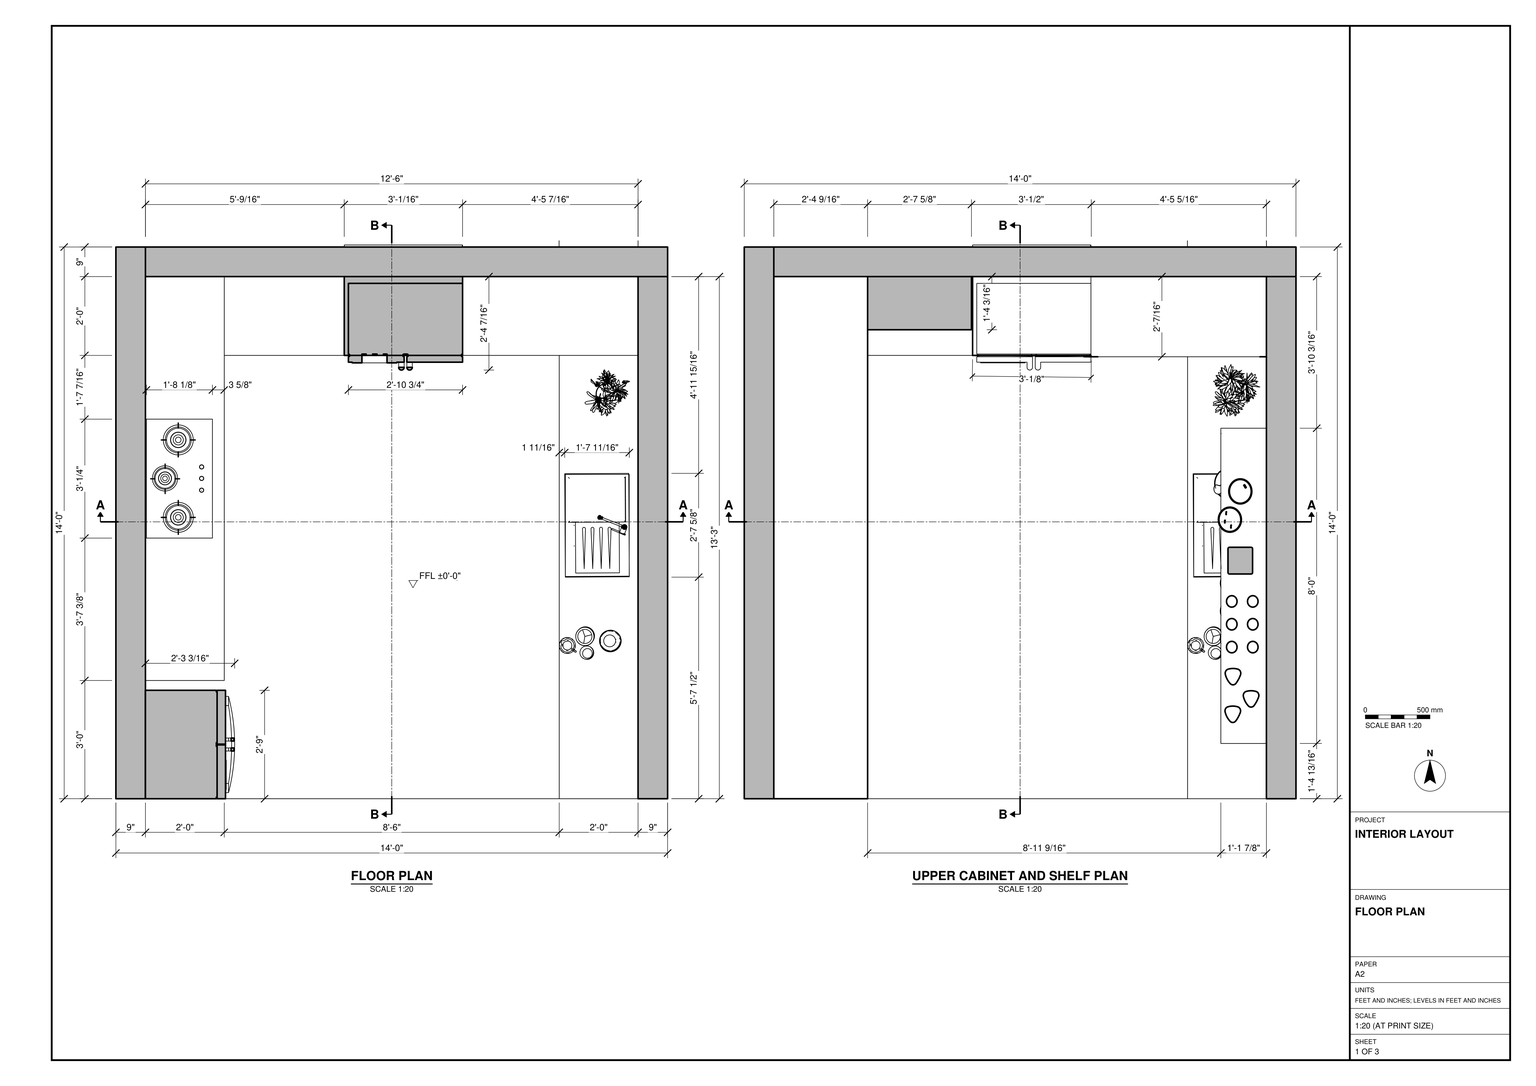
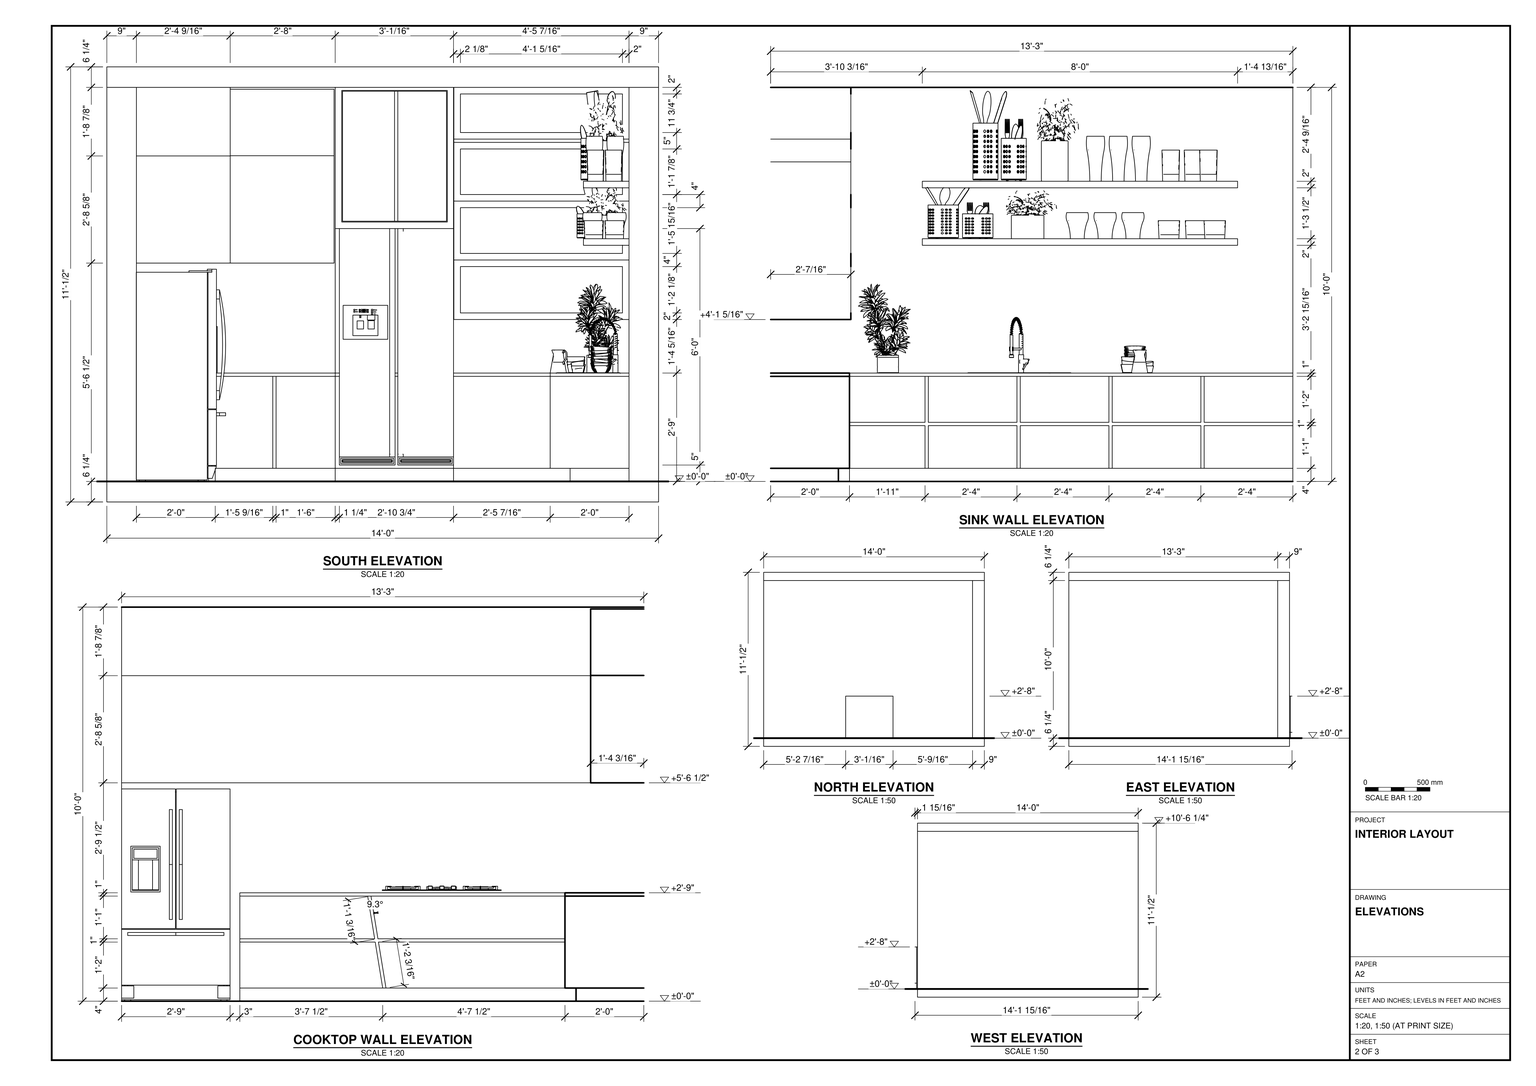
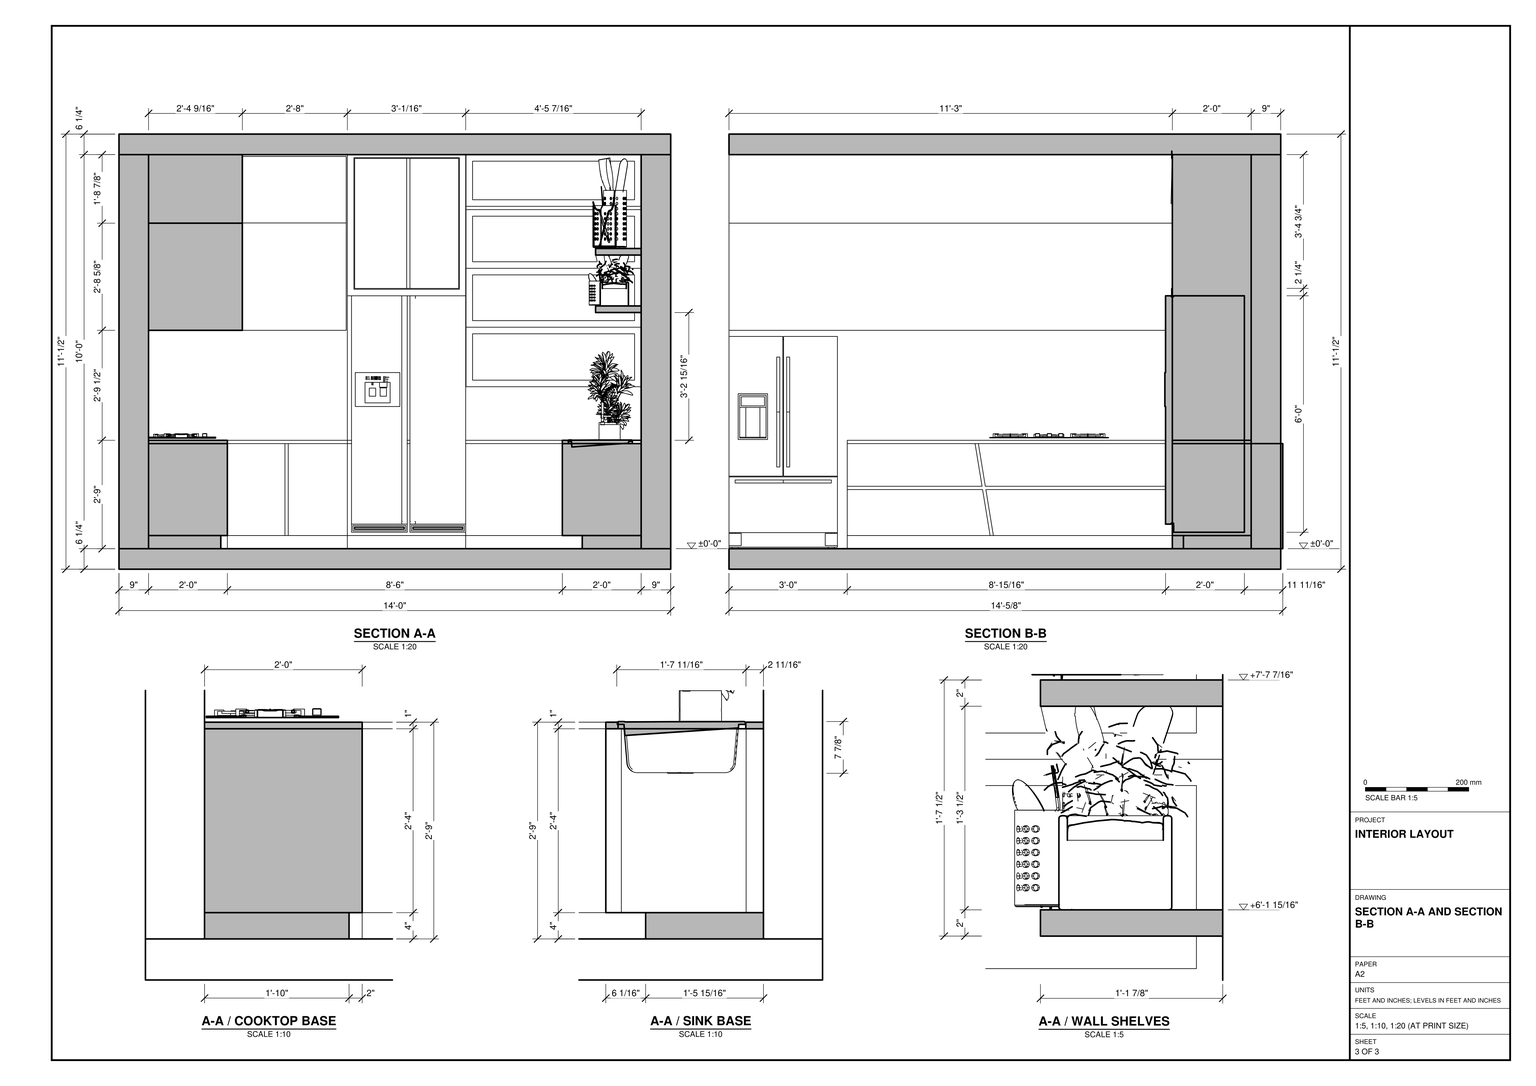
Build the kitchen interior shown in task_files/diagram_01.pdf. Work in feet and inches. The overall model is 14'-0" wide, 14'-5/8" deep and 11'-1/2" high, with a single finished floor level at ±0'-0". Model the floor and ceiling slabs and the 9" side and back walls, leaving the front open as drawn.

Use the floor plan to set out the cooktop run on the left and the sink run on the right, with 8'-6" clear between their counter edges. Use the elevations and section details to shape the worktops, recessed plinths and cabinet fronts. Include the sink, drainer and faucet. Place one refrigerator at the open end of the cooktop wall and the other in the back-wall cabinetry. Follow the upper cabinet and shelf plan for the overhead cupboards and the pair of long shelves above the sink counter. Decor and loose items, including plants, vessels and appliances, may be any suitable library components placed as shown.

Keep the walls and slabs and each piece of joinery or furniture in separate groups or components, and use components for repeated parts. Save one SketchUp model as output_files/kitchen_with_opposing_counters_and_wall_mounted_storage.skp.

# SketchUp Ruby script. Lengths in inches.
U = 1.inch
M = Sketchup.active_model
def pt(a) = Geom::Point3d.new(a.map { |v| v * U })
def face(e, loops, mat)
  f = e.add_face(loops[0].map { |a| pt(a) })
  loops[1..].each { |l| e.add_face(l.map { |a| pt(a) }).erase! }
  f.material = f.back_material = mat if mat
  f
end
# faces: each face lists its corners as indices into pts; further lists are holes
def faces(e, pts, list, mat = nil) = list.each { |f| face(e, (f[0].is_a?(Array) ? f : [f]).map { |l| l.map { |i| pts[i] } }, mat) }
# xy, xz, yz: faces in a plane at the given z, y or x. An outline is a flat list of corners, or four numbers for a rectangle; further outlines are holes
def ring(l) = l.size == 4 ? [[l[0], l[1]], [l[2], l[1]], [l[2], l[3]], [l[0], l[3]]] : l.each_slice(2).to_a
def flat(e, list, mat, &to3) = list.each { |f| face(e, (f[0].is_a?(Array) ? f : [f]).map { |l| ring(l).map { |u, v| to3.(u, v) } }, mat) }
def xy(e, z, list, mat = nil) = flat(e, list, mat) { |x, y| [x, y, z] }
def xz(e, y, list, mat = nil) = flat(e, list, mat) { |x, z| [x, y, z] }
def yz(e, x, list, mat = nil) = flat(e, list, mat) { |y, z| [x, y, z] }
def lines(e, pts, list) = list.each { |a, b| e.add_line(pt(pts[a]), pt(pts[b])) }
# prism: a flat outline (further loops are holes) pulled along v
def prism(e, loops, v, mat = nil)
  f = face(e, loops, mat); d = Geom::Vector3d.new(v.map { |x| x * U })
  f.pushpull(f.normal.samedirection?(d) ? d.length : -d.length)
end
def box(e, o, s, mat = nil) = prism(e, [[o, [o[0] + s[0], o[1], o[2]], [o[0] + s[0], o[1] + s[1], o[2]], [o[0], o[1] + s[1], o[2]]]], [0, 0, s[2]], mat)
def at(x, y, z, deg = 0) = Geom::Transformation.translation(pt([x, y, z])) * Geom::Transformation.rotation(ORIGIN, Z_AXIS, deg.degrees)
def axes(o, x, y, z) = Geom::Transformation.new([*x, 0, *y, 0, *z, 0, *pt(o).to_a, 1])
def part(name) = M.definitions.add(name)
# library, detail: a bought-in or finely detailed component or shape, given as its bounding box
def library(name, o, s) = part(name).tap { |d| box(d.entities, o, s) }
def detail(e, o, s) = box(e.add_group.entities, o, s)
def put(e, d, t, mat = nil) = e.add_instance(d, t).tap { |i| i.material = mat if mat }
def group(e, t, mat = nil) = e.add_group.tap { |g| g.transformation = t; g.material = mat if mat }.entities
root = M.entities
M.materials.add("[Concrete Tile]").color = [203, 190, 164]
M.materials.add("[Field Square Tile]").color = [217, 201, 169]
M.materials.add("[Marble Carrara Gold Floor Tile]").color = [225, 223, 217]
M.materials.add("[Tile Canvas]").color = [199, 192, 173]
M.materials.add("[Tile Ceramic Multi]").color = [165, 115, 84]
M.materials.add("[Wood Square Tile 01]").color = [164, 91, 44]
c1 = library("Fridge\#1",[0,-2.9,-33.83],[42,31.9,87])
c2 = library("French door refrigerator",[0,0,0],[35.5,29.25,69.5])
c3 = library("Kitchen sink",[0,0,0],[31.5,19.49,24.78])
c4 = library("plant",[-35.72,-28.42,0],[66.31,67.39,84.38])
c5 = library("Bosch Stove",[0,0,0],[36.22,20.12,1.38])
c6 = library("3",[-1.02,-0.875,0],[20.82,14.52,8.31])
c7 = library("cups",[-1.65,2.1875,0],[44.23,8.89,10.3125])
c8 = part("Difference")
prism(c8.entities,[[[24,135,0],[24,0,0],[0,0,0],[0,135,0]],[[1.87,67.61,0],[21.31,67.61,0],[21.31,98.77,0],[1.87,98.77,0]]],[0,0,1])
xy(root,6.25,[[69.53,135,105.57,139.0625]])
xy(root,10.25,[[137.36,73.95,156.36,104.95],[69.53,135,105.57,159]])
xy(root,55.5625,[[105.57,134.59,159,159]])
xy(root,78.16,[[145.125,16.82,159,112.82]])
xy(root,80.16,[[145.125,16.82,159,112.82]],"[Tile Ceramic Multi]")
xy(root,95.66,[[145.125,16.82,159,112.82]])
xy(root,97.66,[[145.125,16.82,159,112.82]],"[Tile Ceramic Multi]")
xy(root,126.25,[[105.57,134.59,159,159]])
xz(root,16.82,[[145.125,78.16,159,80.16],[145.125,95.66,159,97.66]])
xz(root,112.82,[[145.125,78.16,159,80.16],[145.125,95.66,159,97.66]])
xz(root,134.59,[[105.57,55.5625,105.67,126.25],[[105.67,55.5625,159,73.6875],[107.67,57.5625,157,71.6875]],[[105.67,73.6875,159,91.625],[107.67,75.6875,157,89.625]],[[105.67,91.625,159,109.5],[107.67,93.625,157,107.5]],[105.67,109.5,159,110.5],
  [[105.67,110.5,159,126.25],[107.67,112.5,157,124.25]]])
xz(root,135,[[69.53,6.25,105.57,10.25]])
xz(root,135,[[69.53,38.25,105.57,126.25]],"[Wood Square Tile 01]")
xz(root,159,[[105.57,55.5625,159,126.25]],"[Wood Square Tile 01]")
yz(root,69.53,[[135,10.25,159,126.25]])
yz(root,105.57,[[135,10.25,159,55.5625],[134.59,55.5625,135,126.25]])
yz(root,145.125,[[16.82,78.16,112.82,80.16],[16.82,95.66,112.82,97.66]])
yz(root,159,[[134.59,55.5625,159,103.5625],[16.82,78.16,112.82,80.16],[16.82,95.66,112.82,97.66],[134.59,103.5625,159,110.5],[134.59,110.5,159,126.25]])
p = [[105.67,134.59,127.32],[69.53,135,127.32],[69.53,135,126.25],[69.53,135,83.25],[105.67,134.59,83.25],[105.67,134.59,91.625],
  [105.67,134.59,109.5],[105.67,134.59,110.5],[105.67,134.59,126.25],[71.53,134.98,85.25],[71.53,134.98,125.32],[103.67,134.61,125.32],
  [103.67,134.61,110.5],[103.67,134.61,109.5],[103.67,134.61,91.625],[103.67,134.61,85.25],[71.77,134.97,85.5],[71.77,134.97,125.08],
  [87.6,134.79,125.08],[103.43,134.61,125.08],[103.43,134.61,85.5],[87.6,134.79,85.5],[159,169.92,38.25],[159,168,38.25],
  [134.95,168,10.69],[134.95,169.92,10.69],[69.53,139.0625,6.25],[69.53,139.0625,10.25],[105.57,139.0625,10.25],[105.57,139.0625,6.25],
  [135,28,38.25],[135,28,24.25],[135,56,38.25],[135,56,24.25],[135,84,38.25],[135,84,24.25],
  [135,112,38.25],[135,112,24.25],[50.54,135,38.25],[50.54,135,10.25],[135,0,24.25],[135,27,24.25],
  [135,55,24.25],[135,83,24.25],[135,111,24.25],[135,135,24.25],[69.53,134.59,111.25],[135,27,38.25],
  [135,55,38.25],[135,112,23.25],[135,135,23.25],[135,28,23.25],[135,55,23.25],[135,56,23.25],
  [135,83,23.25],[135,84,23.25],[135,111,23.25],[135,0,23.25],[135,27,23.25],[135,28,10.25],
  [135,56,10.25],[135,84,10.25],[135,112,10.25],[135,27,10.25],[135,55,10.25],[135,83,38.25],
  [135,83,10.25],[135,111,38.25],[135,111,10.25],[33,74.92,38.25],[33,77.05,25.25],[33,77.21,24.25],
  [33,79.5,10.25],[33,78.21,24.25],[33,80.5,10.25],[33,135,24.25],[33,78.21,25.25],[33,135,25.25],
  [33,75.92,38.25],[33,78.05,25.25],[33,31.57,25.25],[33,31.48,25.25],[51.54,135,38.25],[51.54,135,10.25],
  [88.6,134.79,125.08],[88.6,134.79,85.5],[33,36,24.25],[33,36,25.25],[156.36,104.95,39.25],[156.36,104.95,10.25],
  [156.36,73.95,39.25],[156.36,73.95,10.25],[137.36,104.95,39.25],[137.36,104.95,10.25],[137.36,73.95,39.25],[137.36,73.95,10.25]]
faces(root,p,[[[0,1,2,3,4,5,6,7,8],[9,10,11,12,13,14,15]],[[10,9,15,14,13,12,11],[16,17,18,19,20,21]]])
lines(root,p,[[22,23],[24,25],[26,27],[28,29],[30,31],[32,33],[34,35],[36,37],[38,39],[40,41],[31,42],[33,43],
  [35,44],[37,45],[46,1],[47,41],[48,42],[49,50],[51,52],[53,54],[55,56],[57,58],[51,59],[53,60],
  [55,61],[49,62],[58,63],[52,64],[65,43],[54,66],[67,44],[56,68],[69,70],[71,72],[73,74],[73,75],
  [76,77],[78,79],[76,79],[80,81],[82,83],[18,21],[84,85],[71,86],[70,87],[88,89],[90,91],[92,93],
  [94,95]])
put(root,c1,axes([70.8,132.93,39.25],[0.8277,0,0],[0,0.8277,0],[0,0,0.8277]))
put(root,c2,axes([8.96,33.01,6.25],[0,-0.93,0],[0.93,0,0],[0,0,0.93]))
put(root,c3,at(136.67,98.97,31.47,-89.672))
put(root,c4,axes([149.17,122.76,39.25],[0.3213,0,0],[0,0.3213,0],[0,0,0.3213]))
put(root,c5,at(29.4,79.37,39.95,90))
put(root,c6,at(135,41.36,39.25))
put(root,c7,axes([140.16,98.27,97.66],[0,-1.76715,0],[1.62497,0,0],[0,0,2.6775]))
put(root,c7,axes([138.34,112.14,80.16],[0,-2.15212,0],[1.86391,0,0],[0,0,1.55456]))
g1 = group(root,at(0,0,0),"[Field Square Tile]")
g2 = group(g1,at(0,0,0))
box(g2,[0,0,0],[168,168,6.25])
box(g2,[0,0,126.25],[168,168,6.25])
g3 = group(root,at(0,0,6.25),"[Tile Canvas]")
box(g3,[0,0,0],[9,168,120])
g4 = group(root,at(9,159,6.25),"[Tile Canvas]")
box(g4,[0,0,0],[159,9,120])
g5 = group(root,at(159,0,6.25),"[Marble Carrara Gold Floor Tile]")
box(g5,[0,0,0],[9,159,120])
g6 = group(root,at(9,0,6.25))
box(g6,[0,36,0],[22,123,4])
g7 = group(root,at(9,0,10.25),"[Wood Square Tile 01]")
box(g7,[0,36,0],[24,123,28])
g8 = group(root,at(9,0,38.25),"[Concrete Tile]")
box(g8,[0,36,0],[24,123,1])
g9 = group(root,at(33,135,6.25))
box(g9,[0,3.375,0],[126,20.625,4])
g10 = group(root,at(33,135,10.25),"[Wood Square Tile 01]")
box(g10,[0,0,0],[126,24,28])
g11 = group(root,at(33,0,6.25),"[Wood Square Tile 01]")
xy(g11,0,[[36.53,135,36.53,157.75,72.48,157.75,72.48,168.625,72.57,168.625,72.57,135],[36.53,157.75,72.48,168.625]])
xy(g11,4,[[102,0,126,135]])
xy(g11,32,[[102,0,126,135],[0,135,36.53,159],[36.53,135,72.48,157.75],[72.48,135,72.57,159],[72.57,135,126,159],
  [36.53,157.75,72.48,159],[36.53,159,72.48,168.625],[72.48,159,72.57,168.625]])
xy(g11,33,[[0,135,126,159]])
xz(g11,0,[[102,4,126,32]])
xz(g11,135,[[102,4,126,32],[0,32,36.53,33],[36.53,32,72.48,33],[72.48,32,72.57,33],[72.57,32,126,33]])
xz(g11,159,[[0,32,126,33]])
xz(g11,168.625,[[36.53,0,72.57,32]])
yz(g11,0,[[135,32,159,33]])
yz(g11,36.53,[[135,0,157.75,32],[157.75,0,168.625,32]])
yz(g11,72.57,[[135,0,168.625,32]])
yz(g11,102,[[0,4,135,32]])
yz(g11,126,[[0,4,135,32],[135,32,159,33]])
p = [[72.48,157.75,32],[72.48,157.75,0]]
lines(g11,p,[[0,1]])
g12 = group(root,at(9,0,105.37),"[Wood Square Tile 01]")
box(g12,[0,0,0],[28.5625,159,20.88])
g13 = group(root,at(9,0,72.74),"[Concrete Tile]")
xy(g13,0,[[0,0,28.5625,159],[28.5625,142.8125,60.1875,159]])
xy(g13,32.63,[[0,0,28.5625,159]])
xy(g13,32.7,[[28.5625,142.8125,60.1875,159]])
xy(g13,52.95,[[28.5625,142.8125,60.1875,159]])
xz(g13,0,[[0,0,28.5625,32.63]])
xz(g13,142.8125,[[28.5625,0,60.1875,32.7],[28.5625,32.7,60.1875,52.95]])
xz(g13,159,[[0,0,28.5625,32.63],[28.5625,32.7,60.1875,52.95]])
yz(g13,0,[[0,0,159,32.63]])
yz(g13,28.5625,[[0,0,142.8125,32.63],[142.8125,0,159,32.63],[142.8125,32.63,159,32.7],[142.8125,32.7,159,52.95]])
yz(g13,60.1875,[[142.8125,0,159,32.7],[142.8125,32.7,159,52.95]])
put(root,c8,at(135,0,38.25),"[Concrete Tile]")
g14 = group(root,at(135,0,6.25))
box(g14,[6.0625,0,0],[17.9375,135,4])
